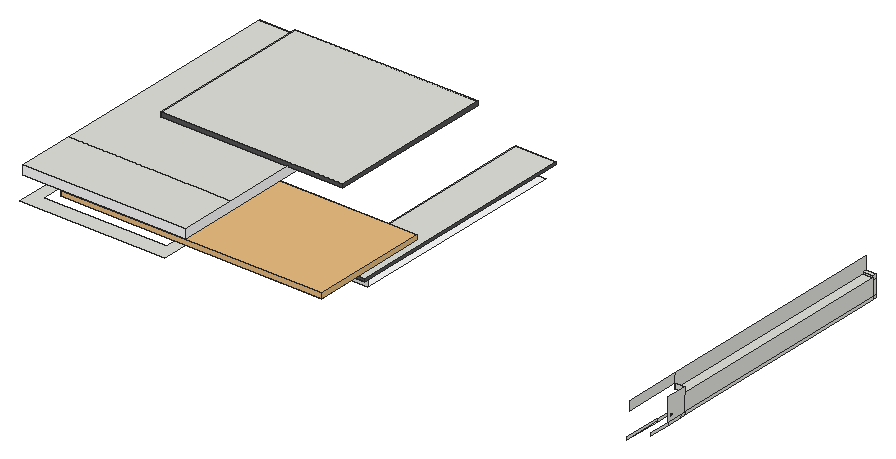
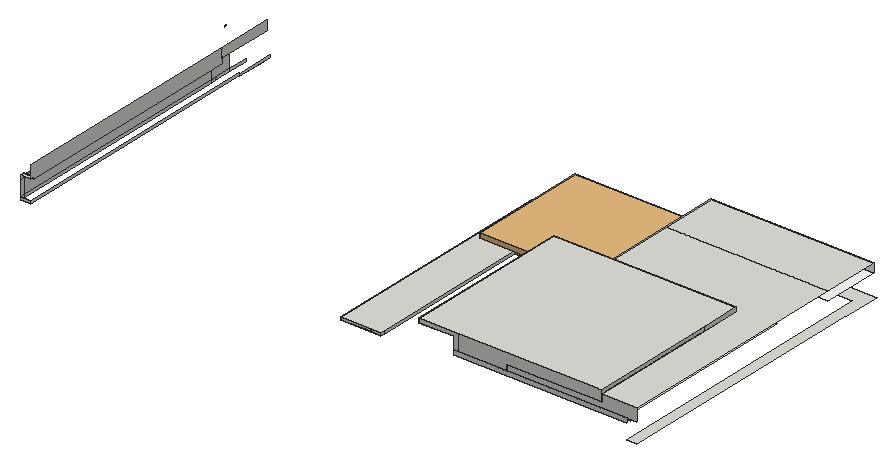
# SketchUp Ruby script. Lengths in inches.
U = 1.inch
M = Sketchup.active_model
def pt(a) = Geom::Point3d.new(a.map { |v| v * U })
def face(e, loops, mat)
  f = e.add_face(loops[0].map { |a| pt(a) })
  loops[1..].each { |l| e.add_face(l.map { |a| pt(a) }).erase! }
  f.material = f.back_material = mat if mat
  f
end
# faces: each face lists its corners as indices into pts; further lists are holes
def faces(e, pts, list, mat = nil) = list.each { |f| face(e, (f[0].is_a?(Array) ? f : [f]).map { |l| l.map { |i| pts[i] } }, mat) }
# xy, xz, yz: faces in a plane at the given z, y or x. An outline is a flat list of corners, or four numbers for a rectangle; further outlines are holes
def ring(l) = l.size == 4 ? [[l[0], l[1]], [l[2], l[1]], [l[2], l[3]], [l[0], l[3]]] : l.each_slice(2).to_a
def flat(e, list, mat, &to3) = list.each { |f| face(e, (f[0].is_a?(Array) ? f : [f]).map { |l| ring(l).map { |u, v| to3.(u, v) } }, mat) }
def xy(e, z, list, mat = nil) = flat(e, list, mat) { |x, y| [x, y, z] }
def xz(e, y, list, mat = nil) = flat(e, list, mat) { |x, z| [x, y, z] }
def yz(e, x, list, mat = nil) = flat(e, list, mat) { |y, z| [x, y, z] }
def lines(e, pts, list) = list.each { |a, b| e.add_line(pt(pts[a]), pt(pts[b])) }
# prism: a flat outline (further loops are holes) pulled along v
def prism(e, loops, v, mat = nil)
  f = face(e, loops, mat); d = Geom::Vector3d.new(v.map { |x| x * U })
  f.pushpull(f.normal.samedirection?(d) ? d.length : -d.length)
end
def box(e, o, s, mat = nil) = prism(e, [[o, [o[0] + s[0], o[1], o[2]], [o[0] + s[0], o[1] + s[1], o[2]], [o[0], o[1] + s[1], o[2]]]], [0, 0, s[2]], mat)
def at(x, y, z, deg = 0) = Geom::Transformation.translation(pt([x, y, z])) * Geom::Transformation.rotation(ORIGIN, Z_AXIS, deg.degrees)
def axes(o, x, y, z) = Geom::Transformation.new([*x, 0, *y, 0, *z, 0, *pt(o).to_a, 1])
def part(name) = M.definitions.add(name)
# library, detail: a bought-in or finely detailed component or shape, given as its bounding box
def library(name, o, s) = part(name).tap { |d| box(d.entities, o, s) }
def detail(e, o, s) = box(e.add_group.entities, o, s)
def put(e, d, t, mat = nil) = e.add_instance(d, t).tap { |i| i.material = mat if mat }
def group(e, t, mat = nil) = e.add_group.tap { |g| g.transformation = t; g.material = mat if mat }.entities
root = M.entities
M.materials.add("[Color M00]").color = [255, 255, 255]
M.materials.add("[Color M06]").color = [86, 86, 86]
c1 = library("Mesh Light\#4",[-0.5,-0.5,-0.1],[1,1,0.2])
c2 = part("Group\#24")
xy(c2.entities,0,[[203.13,95.41,201.58,95.62,200.13,96.22,198.89,97.17,197.9375,98.41,197.34,99.86,197.13,101.41,197.34,102.96,197.9375,104.41,198.89,105.65,200.13,106.61,201.58,107.21,203.13,107.41,204.6875,107.21,206.13,106.61,207.375,105.65,208.33,104.41,208.93,102.96,209.13,101.41,208.93,99.86,208.33,98.41,207.375,97.17,206.13,96.22,204.6875,95.62],[281.57,95.41,280.02,95.62,278.57,96.22,277.33,97.17,276.375,98.41,275.77,99.86,275.57,101.41,275.77,102.96,276.375,104.41,277.33,105.65,278.57,106.61,280.02,107.21,281.57,107.41,283.125,107.21,284.57,106.61,285.8125,105.65,286.77,104.41,287.37,102.96,287.57,101.41,287.37,99.86,286.77,98.41,285.8125,97.17,284.57,96.22,283.125,95.62],[350.95,95.41,349.39,95.62,347.95,96.22,346.7,97.17,345.75,98.41,345.15,99.86,344.95,101.41,345.15,102.96,345.75,104.41,346.7,105.65,347.95,106.61,349.39,107.21,350.95,107.41,352.5,107.21,353.95,106.61,355.1875,105.65,356.14,104.41,356.74,102.96,356.95,101.41,356.74,99.86,356.14,98.41,355.1875,97.17,353.95,96.22,352.5,95.62],[376,162.85,374.44,163.05,373,163.65,371.75,164.6,370.8,165.85,370.2,167.29,370,168.85,370.2,170.4,370.8,171.85,371.75,173.09,373,174.04,374.44,174.64,376,174.85,377.55,174.64,379,174.04,380.24,173.09,381.19,171.85,381.79,170.4,382,168.85,381.79,167.29,381.19,165.85,380.24,164.6,379,163.65,377.55,163.05]],"[Color M00]")
xy(c2.entities,33.4375,[[6,0,4.45,0.2,3,0.8,1.76,1.76,0.8,3,0.2,4.45,0,6,0.2,7.55,0.8,9,1.76,10.24,3,11.2,4.45,11.8,6,12,7.55,11.8,9,11.2,10.24,10.24,11.2,9,11.8,7.55,12,6,11.8,4.45,11.2,3,10.24,1.76,9,0.8,7.55,0.2],[83.125,0,81.57,0.2,80.125,0.8,78.88,1.76,77.93,3,77.33,4.45,77.125,6,77.33,7.55,77.93,9,78.88,10.24,80.125,11.2,81.57,11.8,83.125,12,84.68,11.8,86.125,11.2,87.37,10.24,88.32,9,88.92,7.55,89.125,6,88.92,4.45,88.32,3,87.37,1.76,86.125,0.8,84.68,0.2],[166.6875,0,165.13,0.2,163.6875,0.8,162.44,1.76,161.49,3,160.89,4.45,160.6875,6,160.89,7.55,161.49,9,162.44,10.24,163.6875,11.2,165.13,11.8,166.6875,12,168.24,11.8,169.6875,11.2,170.93,10.24,171.88,9,172.48,7.55,172.6875,6,172.48,4.45,171.88,3,170.93,1.76,169.6875,0.8,168.24,0.2],[166.6875,88.9375,165.13,89.14,163.6875,89.74,162.44,90.69,161.49,91.9375,160.89,93.38,160.6875,94.9375,160.89,96.49,161.49,97.9375,162.44,99.18,163.6875,100.13,165.13,100.73,166.6875,100.9375,168.24,100.73,169.6875,100.13,170.93,99.18,171.88,97.9375,172.48,96.49,172.6875,94.9375,172.48,93.38,171.88,91.9375,170.93,90.69,169.6875,89.74,168.24,89.14]],"[Color M00]")
put(c2.entities,c1,axes([191,87.42,16.72],[382.99758,0,0],[0,175.84579,0],[0,0,34.4375]))
c3 = library("Group\#23",[-0.5,-0.5,-0.1],[13,110.375,0.2])
xy(root,269.375,[[1170.95,584.06,1383.39,584.06,1383.39,676.67,1376.89,676.67,1376.89,706.17,1367.875,706.17,1367.875,607.33,1187.0625,607.33,1187.0625,1021.31,1172.33,1021.31,1172.33,638.99,1170.95,638.99],[1376.89,676.67,1383.39,731.24]])
xy(root,269.375,[[[1383.39,676.67,1383.39,731.24,1567.08,731.24,1567.08,1001.66,1607.7,1001.66,1607.7,676.67],[1497.04,698.72,1498.6,698.92,1500.04,699.52,1501.29,700.47,1502.24,701.72,1502.84,703.16,1503.04,704.72,1502.84,706.27,1502.24,707.72,1501.29,708.96,1500.04,709.91,1498.6,710.51,1497.04,710.72,1495.49,710.51,1494.04,709.91,1492.8,708.96,1491.85,707.72,1491.25,706.27,1491.04,704.72,1491.25,703.16,1491.85,701.72,1492.8,700.47,1494.04,699.52,1495.49,698.92],[1566.42,698.72,1567.97,698.92,1569.42,699.52,1570.66,700.47,1571.61,701.72,1572.21,703.16,1572.42,704.72,1572.21,706.27,1571.61,707.72,1570.66,708.96,1569.42,709.91,1567.97,710.51,1566.42,710.72,1564.86,710.51,1563.42,709.91,1562.17,708.96,1561.22,707.72,1560.62,706.27,1560.42,704.72,1560.62,703.16,1561.22,701.72,1562.17,700.47,1563.42,699.52,1564.86,698.92],[1418.61,698.72,1420.16,698.92,1421.61,699.52,1422.85,700.47,1423.8,701.72,1424.4,703.16,1424.61,704.72,1424.4,706.27,1423.8,707.72,1422.85,708.96,1421.61,709.91,1420.16,710.51,1418.61,710.72,1417.05,710.51,1415.61,709.91,1414.36,708.96,1413.41,707.72,1412.81,706.27,1412.61,704.72,1412.81,703.16,1413.41,701.72,1414.36,700.47,1415.61,699.52,1417.05,698.92],[1591.47,766.15,1593.02,766.35,1594.47,766.95,1595.71,767.91,1596.67,769.15,1597.27,770.6,1597.47,772.15,1597.27,773.7,1596.67,775.15,1595.71,776.39,1594.47,777.35,1593.02,777.95,1591.47,778.15,1589.92,777.95,1588.47,777.35,1587.23,776.39,1586.27,775.15,1585.67,773.7,1585.47,772.15,1585.67,770.6,1586.27,769.15,1587.23,767.91,1588.47,766.95,1589.92,766.35],[1591.47,846.59,1593.02,846.79,1594.47,847.39,1595.71,848.35,1596.67,849.59,1597.27,851.04,1597.47,852.59,1597.27,854.14,1596.67,855.59,1595.71,856.83,1594.47,857.78,1593.02,858.38,1591.47,858.59,1589.92,858.38,1588.47,857.78,1587.23,856.83,1586.27,855.59,1585.67,854.14,1585.47,852.59,1585.67,851.04,1586.27,849.59,1587.23,848.35,1588.47,847.39,1589.92,846.79],[1591.47,943.96,1593.02,944.17,1594.47,944.77,1595.71,945.72,1596.67,946.96,1597.27,948.41,1597.47,949.96,1597.27,951.52,1596.67,952.96,1595.71,954.21,1594.47,955.16,1593.02,955.76,1591.47,955.96,1589.92,955.76,1588.47,955.16,1587.23,954.21,1586.27,952.96,1585.67,951.52,1585.47,949.96,1585.67,948.41,1586.27,946.96,1587.23,945.72,1588.47,944.77,1589.92,944.17]]],"[Color M00]")
xy(root,270.375,[[2063.54,592.75,2064.92,636.6875]])
xy(root,279.25,[[1376.89,670.42,1607.7,676.67],[1376.89,676.67,1376.89,776.62,1548.25,776.62,1548.25,1021.31,1607.7,1021.31,1607.7,676.67]])
xy(root,282.6875,[[1376.89,670.42,1607.7,670.42,1607.7,1021.31,1548.25,1021.31,1548.25,776.62,1376.89,776.62]])
xy(root,291.125,[[1197.375,733.75,1197.375,1014.93,1364.27,1014.93,1364.27,854.49,1354.74,854.49,1354.74,733.75],[1364.27,854.49,1434.7,1014.93]])
xy(root,297.875,[[1187.0625,1014.93,1364.27,1021.31],[1364.27,1014.93,1434.7,1021.31]])
xy(root,299.625,[[2064.92,668.18,2079.65,1012.63]])
xy(root,302.5625,[[2064.92,1012.63,2079.65,1019]])
xy(root,302.8125,[[[1172.33,587.17,1172.33,670.48,1187.0625,670.48,1187.0625,639.17,1364.27,639.17,1364.27,832.12,1410.7,832.12,1410.7,587.17],[1221.47,603.3,1223.03,603.51,1224.47,604.11,1225.71,605.0625,1226.67,606.3,1227.27,607.75,1227.47,609.3,1227.27,610.86,1226.67,612.3,1225.71,613.55,1224.47,614.5,1223.03,615.1,1221.47,615.3,1219.92,615.1,1218.47,614.5,1217.23,613.55,1216.28,612.3,1215.68,610.86,1215.47,609.3,1215.68,607.75,1216.28,606.3,1217.23,605.0625,1218.47,604.11,1219.92,603.51],[1298.6,603.3,1300.15,603.51,1301.6,604.11,1302.84,605.0625,1303.79,606.3,1304.39,607.75,1304.6,609.3,1304.39,610.86,1303.79,612.3,1302.84,613.55,1301.6,614.5,1300.15,615.1,1298.6,615.3,1297.04,615.1,1295.6,614.5,1294.35,613.55,1293.4,612.3,1292.8,610.86,1292.6,609.3,1292.8,607.75,1293.4,606.3,1294.35,605.0625,1295.6,604.11,1297.04,603.51],[1382.16,692.24,1383.71,692.45,1385.16,693.05,1386.4,694,1387.36,695.24,1387.96,696.6875,1388.16,698.24,1387.96,699.8,1387.36,701.24,1386.4,702.48,1385.16,703.4375,1383.71,704.04,1382.16,704.24,1380.61,704.04,1379.16,703.4375,1377.92,702.48,1376.96,701.24,1376.36,699.8,1376.16,698.24,1376.36,696.6875,1376.96,695.24,1377.92,694,1379.16,693.05,1380.61,692.45],[1382.16,603.3,1383.71,603.51,1385.16,604.11,1386.4,605.0625,1387.36,606.3,1387.96,607.75,1388.16,609.3,1387.96,610.86,1387.36,612.3,1386.4,613.55,1385.16,614.5,1383.71,615.1,1382.16,615.3,1380.61,615.1,1379.16,614.5,1377.92,613.55,1376.96,612.3,1376.36,610.86,1376.16,609.3,1376.36,607.75,1376.96,606.3,1377.92,605.0625,1379.16,604.11,1380.61,603.51]]],"[Color M00]")
xy(root,305.625,[[1224.7,832.12,1364.27,1021.31]])
xy(root,316.0625,[[1172.33,587.17,1410.7,670.48],[1172.33,670.48,1410.7,670.48,1410.7,774.49,1224.7,774.49,1224.7,1021.31,1172.33,1021.31],[1410.7,774.49,1410.7,832.12,1440.7,832.12,1440.7,1021.31,1492.27,1021.31,1492.27,774.49]])
xy(root,321.8125,[[1224.7,774.49,1492.27,1021.31]])
xz(root,587.17,[[1172.33,302.8125,1410.7,316.0625]],"[Color M00]")
xz(root,636.6875,[[2063.54,270.375,2064.92,274.0625]])
xz(root,668.18,[[2064.92,299.625,2079.65,307.5]])
xz(root,670.42,[[1376.89,279.25,1607.7,282.6875]],"[Color M06]")
xz(root,676.67,[[1376.89,269.375,1607.7,279.25]])
xz(root,774.49,[[1224.7,316.0625,1492.27,321.8125]],"[Color M06]")
xz(root,776.62,[[1376.89,279.25,1548.25,282.6875]])
xz(root,832.12,[[1364.27,302.8125,1410.7,305.625]])
xz(root,1012.63,[[2064.92,299.625,2079.65,302.5625]])
xz(root,1014.93,[[1187.0625,291.125,1364.27,297.875],[1364.27,291.125,1434.7,297.875]])
xz(root,1019,[[2064.92,270.375,2079.65,274.0625]])
xz(root,1021.31,[[1548.25,279.25,1563.95,282.6875],[1563.95,279.25,1607.7,282.6875],[1187.0625,291.125,1440.7,297.875],[1172.33,297.875,1172.33,316.0625,1224.7,316.0625,1224.7,305.625,1364.27,305.625,1364.27,297.875],[1364.27,297.875,1364.27,305.625,1224.7,305.625,1224.7,321.8125,1434.7,321.8125,1434.7,297.875],
  [1434.7,297.875,1434.7,321.8125,1492.27,321.8125,1492.27,316.0625,1440.7,316.0625,1440.7,297.875]])
yz(root,1224.7,[[804.12,305.625,832.12,316.0625],[832.12,305.625,1021.31,316.0625],[774.49,316.0625,832.12,321.8125],[832.12,316.0625,1021.31,321.8125]])
yz(root,1364.27,[[832.12,291.125,1014.93,297.875],[832.12,297.875,1021.31,305.625]])
yz(root,1376.89,[[670.42,279.25,776.62,282.6875]])
yz(root,1410.7,[[587.17,302.8125,832.12,316.0625]],"[Color M00]")
yz(root,1492.27,[[774.49,316.0625,1021.31,321.8125]],"[Color M06]")
yz(root,1548.25,[[776.62,279.25,1014.93,282.6875],[1014.93,279.25,1021.31,282.6875]])
yz(root,1607.7,[[670.42,279.25,1021.31,282.6875]],"[Color M06]")
yz(root,2063.54,[[581.75,270.375,636.6875,274.0625]])
yz(root,2064.92,[[636.6875,270.375,1019,274.0625],[668.18,299.625,668.18,320.75,1019,320.75,1019,302.5625,1012.63,302.5625,1012.63,299.625],[584.86,307.5,668.18,320.75]])
yz(root,2079.65,[[605.03,270.375,636.86,274.0625],[636.86,270.375,660.21,274.0625],[660.21,270.375,668.18,274.0625],[668.18,270.375,1012.63,274.0625],[1012.63,270.375,1019,274.0625],
  [636.86,274.0625,668.18,307.5],[668.18,274.0625,1012.63,299.625],[1012.63,274.0625,1019,295.8125],[1012.63,295.8125,1019,302.5625]])
p = [[1418.61,698.72,269.375],[1417.05,698.92,269.375],[1417.05,698.92,270.0625],[1418.61,698.72,270.0625],[1420.16,698.92,269.375],[1420.16,698.92,270.0625],
  [1497.04,698.72,269.375],[1495.49,698.92,269.375],[1495.49,698.92,270.0625],[1497.04,698.72,270.0625],[1498.6,698.92,269.375],[1498.6,698.92,270.0625],
  [1566.42,698.72,269.375],[1564.86,698.92,269.375],[1564.86,698.92,270.0625],[1566.42,698.72,270.0625],[1567.97,698.92,269.375],[1567.97,698.92,270.0625],
  [1415.61,699.52,269.375],[1415.61,699.52,270.0625],[1421.61,699.52,269.375],[1421.61,699.52,270.0625],[1494.04,699.52,269.375],[1494.04,699.52,270.0625],
  [1500.04,699.52,269.375],[1500.04,699.52,270.0625],[1563.42,699.52,269.375],[1563.42,699.52,270.0625],[1569.42,699.52,269.375],[1569.42,699.52,270.0625],
  [1414.36,700.47,269.375],[1414.36,700.47,270.0625],[1422.85,700.47,269.375],[1422.85,700.47,270.0625],[1492.8,700.47,269.375],[1492.8,700.47,270.0625],
  [1501.29,700.47,269.375],[1501.29,700.47,270.0625],[1562.17,700.47,269.375],[1562.17,700.47,270.0625],[1570.66,700.47,269.375],[1570.66,700.47,270.0625],
  [1413.41,701.72,269.375],[1413.41,701.72,270.0625],[1423.8,701.72,269.375],[1423.8,701.72,270.0625],[1491.85,701.72,269.375],[1491.85,701.72,270.0625],
  [1502.24,701.72,269.375],[1502.24,701.72,270.0625],[1561.22,701.72,269.375],[1561.22,701.72,270.0625],[1571.61,701.72,269.375],[1571.61,701.72,270.0625],
  [1412.81,703.16,269.375],[1412.81,703.16,270.0625],[1424.4,703.16,269.375],[1424.4,703.16,270.0625],[1491.25,703.16,269.375],[1491.25,703.16,270.0625],
  [1502.84,703.16,269.375],[1502.84,703.16,270.0625],[1560.62,703.16,269.375],[1560.62,703.16,270.0625],[1572.21,703.16,269.375],[1572.21,703.16,270.0625],
  [1412.61,704.72,269.375],[1412.61,704.72,270.0625],[1424.61,704.72,269.375],[1424.61,704.72,270.0625],[1491.04,704.72,269.375],[1491.04,704.72,270.0625],
  [1503.04,704.72,269.375],[1503.04,704.72,270.0625],[1560.42,704.72,269.375],[1560.42,704.72,270.0625],[1572.42,704.72,269.375],[1572.42,704.72,270.0625],
  [1412.81,706.27,269.375],[1412.81,706.27,270.0625],[1424.4,706.27,269.375],[1424.4,706.27,270.0625],[1491.25,706.27,269.375],[1491.25,706.27,270.0625],
  [1502.84,706.27,269.375],[1502.84,706.27,270.0625],[1560.62,706.27,269.375],[1560.62,706.27,270.0625],[1572.21,706.27,269.375],[1572.21,706.27,270.0625],
  [1413.41,707.72,269.375],[1413.41,707.72,270.0625],[1423.8,707.72,269.375],[1423.8,707.72,270.0625],[1491.85,707.72,269.375],[1491.85,707.72,270.0625],
  [1502.24,707.72,269.375],[1502.24,707.72,270.0625],[1561.22,707.72,269.375],[1561.22,707.72,270.0625],[1571.61,707.72,269.375],[1571.61,707.72,270.0625],
  [1414.36,708.96,269.375],[1414.36,708.96,270.0625],[1422.85,708.96,269.375],[1422.85,708.96,270.0625],[1492.8,708.96,269.375],[1492.8,708.96,270.0625],
  [1501.29,708.96,269.375],[1501.29,708.96,270.0625],[1562.17,708.96,269.375],[1562.17,708.96,270.0625],[1570.66,708.96,269.375],[1570.66,708.96,270.0625],
  [1415.61,709.91,269.375],[1415.61,709.91,270.0625],[1421.61,709.91,269.375],[1421.61,709.91,270.0625],[1494.04,709.91,269.375],[1494.04,709.91,270.0625],
  [1500.04,709.91,269.375],[1500.04,709.91,270.0625],[1563.42,709.91,269.375],[1563.42,709.91,270.0625],[1569.42,709.91,269.375],[1569.42,709.91,270.0625],
  [1417.05,710.51,269.375],[1417.05,710.51,270.0625],[1420.16,710.51,269.375],[1420.16,710.51,270.0625],[1495.49,710.51,269.375],[1495.49,710.51,270.0625],
  [1498.6,710.51,269.375],[1498.6,710.51,270.0625],[1564.86,710.51,269.375],[1564.86,710.51,270.0625],[1567.97,710.51,269.375],[1567.97,710.51,270.0625],
  [1418.61,710.72,269.375],[1418.61,710.72,270.0625],[1497.04,710.72,269.375],[1497.04,710.72,270.0625],[1566.42,710.72,269.375],[1566.42,710.72,270.0625],
  [1591.47,766.15,269.375],[1589.92,766.35,269.375],[1589.92,766.35,270.0625],[1591.47,766.15,270.0625],[1593.02,766.35,269.375],[1593.02,766.35,270.0625],
  [1588.47,766.95,269.375],[1588.47,766.95,270.0625],[1594.47,766.95,269.375],[1594.47,766.95,270.0625],[1587.23,767.91,269.375],[1587.23,767.91,270.0625],
  [1595.71,767.91,269.375],[1595.71,767.91,270.0625],[1586.27,769.15,269.375],[1586.27,769.15,270.0625],[1596.67,769.15,269.375],[1596.67,769.15,270.0625],
  [1585.67,770.6,269.375],[1585.67,770.6,270.0625],[1597.27,770.6,269.375],[1597.27,770.6,270.0625],[1585.47,772.15,269.375],[1585.47,772.15,270.0625],
  [1597.47,772.15,269.375],[1597.47,772.15,270.0625],[1585.67,773.7,269.375],[1585.67,773.7,270.0625],[1597.27,773.7,269.375],[1597.27,773.7,270.0625],
  [1586.27,775.15,269.375],[1586.27,775.15,270.0625],[1596.67,775.15,269.375],[1596.67,775.15,270.0625],[1587.23,776.39,269.375],[1587.23,776.39,270.0625],
  [1595.71,776.39,269.375],[1595.71,776.39,270.0625],[1588.47,777.35,269.375],[1588.47,777.35,270.0625],[1594.47,777.35,269.375],[1594.47,777.35,270.0625],
  [1589.92,777.95,269.375],[1589.92,777.95,270.0625],[1593.02,777.95,269.375],[1593.02,777.95,270.0625],[1591.47,778.15,269.375],[1591.47,778.15,270.0625],
  [1591.47,846.59,269.375],[1589.92,846.79,269.375],[1589.92,846.79,270.0625],[1591.47,846.59,270.0625],[1593.02,846.79,269.375],[1593.02,846.79,270.0625],
  [1588.47,847.39,269.375],[1588.47,847.39,270.0625],[1594.47,847.39,269.375],[1594.47,847.39,270.0625],[1587.23,848.35,269.375],[1587.23,848.35,270.0625],
  [1595.71,848.35,269.375],[1595.71,848.35,270.0625],[1586.27,849.59,269.375],[1586.27,849.59,270.0625],[1596.67,849.59,269.375],[1596.67,849.59,270.0625],
  [1585.67,851.04,269.375],[1585.67,851.04,270.0625],[1597.27,851.04,269.375],[1597.27,851.04,270.0625],[1585.47,852.59,269.375],[1585.47,852.59,270.0625],
  [1597.47,852.59,269.375],[1597.47,852.59,270.0625],[1585.67,854.14,269.375],[1585.67,854.14,270.0625],[1597.27,854.14,269.375],[1597.27,854.14,270.0625],
  [1586.27,855.59,269.375],[1586.27,855.59,270.0625],[1596.67,855.59,269.375],[1596.67,855.59,270.0625],[1587.23,856.83,269.375],[1587.23,856.83,270.0625],
  [1595.71,856.83,269.375],[1595.71,856.83,270.0625],[1588.47,857.78,269.375],[1588.47,857.78,270.0625],[1594.47,857.78,269.375],[1594.47,857.78,270.0625],
  [1589.92,858.38,269.375],[1589.92,858.38,270.0625],[1593.02,858.38,269.375],[1593.02,858.38,270.0625],[1591.47,858.59,269.375],[1591.47,858.59,270.0625],
  [1591.47,943.96,269.375],[1589.92,944.17,269.375],[1589.92,944.17,270.0625],[1591.47,943.96,270.0625],[1593.02,944.17,269.375],[1593.02,944.17,270.0625],
  [1588.47,944.77,269.375],[1588.47,944.77,270.0625],[1594.47,944.77,269.375],[1594.47,944.77,270.0625],[1587.23,945.72,269.375],[1587.23,945.72,270.0625],
  [1595.71,945.72,269.375],[1595.71,945.72,270.0625],[1586.27,946.96,269.375],[1586.27,946.96,270.0625],[1596.67,946.96,269.375],[1596.67,946.96,270.0625],
  [1585.67,948.41,269.375],[1585.67,948.41,270.0625],[1597.27,948.41,269.375],[1597.27,948.41,270.0625],[1585.47,949.96,269.375],[1585.47,949.96,270.0625],
  [1597.47,949.96,269.375],[1597.47,949.96,270.0625],[1585.67,951.52,269.375],[1585.67,951.52,270.0625],[1597.27,951.52,269.375],[1597.27,951.52,270.0625],
  [1586.27,952.96,269.375],[1586.27,952.96,270.0625],[1596.67,952.96,269.375],[1596.67,952.96,270.0625],[1587.23,954.21,269.375],[1587.23,954.21,270.0625],
  [1595.71,954.21,269.375],[1595.71,954.21,270.0625],[1588.47,955.16,269.375],[1588.47,955.16,270.0625],[1594.47,955.16,269.375],[1594.47,955.16,270.0625],
  [1589.92,955.76,269.375],[1589.92,955.76,270.0625],[1593.02,955.76,269.375],[1593.02,955.76,270.0625],[1591.47,955.96,269.375],[1591.47,955.96,270.0625],
  [1221.47,603.3,302.8125],[1219.92,603.51,302.8125],[1219.92,603.51,303.5],[1221.47,603.3,303.5],[1223.03,603.51,302.8125],[1223.03,603.51,303.5],
  [1298.6,603.3,302.8125],[1297.04,603.51,302.8125],[1297.04,603.51,303.5],[1298.6,603.3,303.5],[1300.15,603.51,302.8125],[1300.15,603.51,303.5],
  [1382.16,603.3,302.8125],[1380.61,603.51,302.8125],[1380.61,603.51,303.5],[1382.16,603.3,303.5],[1383.71,603.51,302.8125],[1383.71,603.51,303.5],
  [1218.47,604.11,302.8125],[1218.47,604.11,303.5],[1224.47,604.11,302.8125],[1224.47,604.11,303.5],[1295.6,604.11,302.8125],[1295.6,604.11,303.5],
  [1301.6,604.11,302.8125],[1301.6,604.11,303.5],[1379.16,604.11,302.8125],[1379.16,604.11,303.5],[1385.16,604.11,302.8125],[1385.16,604.11,303.5],
  [1217.23,605.0625,302.8125],[1217.23,605.0625,303.5],[1225.71,605.0625,302.8125],[1225.71,605.0625,303.5],[1294.35,605.0625,302.8125],[1294.35,605.0625,303.5],
  [1302.84,605.0625,302.8125],[1302.84,605.0625,303.5],[1377.92,605.0625,302.8125],[1377.92,605.0625,303.5],[1386.4,605.0625,302.8125],[1386.4,605.0625,303.5],
  [1216.28,606.3,302.8125],[1216.28,606.3,303.5],[1226.67,606.3,302.8125],[1226.67,606.3,303.5],[1293.4,606.3,302.8125],[1293.4,606.3,303.5],
  [1303.79,606.3,302.8125],[1303.79,606.3,303.5],[1376.96,606.3,302.8125],[1376.96,606.3,303.5],[1387.36,606.3,302.8125],[1387.36,606.3,303.5],
  [1215.68,607.75,302.8125],[1215.68,607.75,303.5],[1227.27,607.75,302.8125],[1227.27,607.75,303.5],[1292.8,607.75,302.8125],[1292.8,607.75,303.5],
  [1304.39,607.75,302.8125],[1304.39,607.75,303.5],[1376.36,607.75,302.8125],[1376.36,607.75,303.5],[1387.96,607.75,302.8125],[1387.96,607.75,303.5],
  [1227.47,609.3,302.8125],[1227.47,609.3,303.5],[1292.6,609.3,302.8125],[1292.6,609.3,303.5],[1304.6,609.3,302.8125],[1304.6,609.3,303.5],
  [1376.16,609.3,302.8125],[1376.16,609.3,303.5],[1388.16,609.3,302.8125],[1388.16,609.3,303.5],[1215.47,609.3,302.8125],[1215.68,610.86,302.8125],
  [1215.68,610.86,303.5],[1215.47,609.3,303.5],[1227.27,610.86,302.8125],[1227.27,610.86,303.5],[1292.8,610.86,302.8125],[1292.8,610.86,303.5],
  [1304.39,610.86,302.8125],[1304.39,610.86,303.5],[1376.36,610.86,302.8125],[1376.36,610.86,303.5],[1387.96,610.86,302.8125],[1387.96,610.86,303.5],
  [1216.28,612.3,302.8125],[1216.28,612.3,303.5],[1226.67,612.3,302.8125],[1226.67,612.3,303.5],[1293.4,612.3,302.8125],[1293.4,612.3,303.5],
  [1303.79,612.3,302.8125],[1303.79,612.3,303.5],[1376.96,612.3,302.8125],[1376.96,612.3,303.5],[1387.36,612.3,302.8125],[1387.36,612.3,303.5],
  [1217.23,613.55,302.8125],[1217.23,613.55,303.5],[1225.71,613.55,302.8125],[1225.71,613.55,303.5],[1294.35,613.55,302.8125],[1294.35,613.55,303.5],
  [1302.84,613.55,302.8125],[1302.84,613.55,303.5],[1377.92,613.55,302.8125],[1377.92,613.55,303.5],[1386.4,613.55,302.8125],[1386.4,613.55,303.5],
  [1218.47,614.5,302.8125],[1218.47,614.5,303.5],[1224.47,614.5,302.8125],[1224.47,614.5,303.5],[1295.6,614.5,302.8125],[1295.6,614.5,303.5],
  [1301.6,614.5,302.8125],[1301.6,614.5,303.5],[1379.16,614.5,302.8125],[1379.16,614.5,303.5],[1385.16,614.5,302.8125],[1385.16,614.5,303.5],
  [1219.92,615.1,302.8125],[1219.92,615.1,303.5],[1223.03,615.1,302.8125],[1223.03,615.1,303.5],[1297.04,615.1,302.8125],[1297.04,615.1,303.5],
  [1300.15,615.1,302.8125],[1300.15,615.1,303.5],[1380.61,615.1,302.8125],[1380.61,615.1,303.5],[1383.71,615.1,302.8125],[1383.71,615.1,303.5],
  [1221.47,615.3,302.8125],[1221.47,615.3,303.5],[1298.6,615.3,302.8125],[1298.6,615.3,303.5],[1382.16,615.3,302.8125],[1382.16,615.3,303.5],
  [1382.16,692.24,302.8125],[1380.61,692.45,302.8125],[1380.61,692.45,303.5],[1382.16,692.24,303.5],[1383.71,692.45,302.8125],[1383.71,692.45,303.5],
  [1379.16,693.05,302.8125],[1379.16,693.05,303.5],[1385.16,693.05,302.8125],[1385.16,693.05,303.5],[1377.92,694,302.8125],[1377.92,694,303.5],
  [1386.4,694,302.8125],[1386.4,694,303.5],[1376.96,695.24,302.8125],[1376.96,695.24,303.5],[1387.36,695.24,302.8125],[1387.36,695.24,303.5],
  [1376.36,696.6875,302.8125],[1376.36,696.6875,303.5],[1387.96,696.6875,302.8125],[1387.96,696.6875,303.5],[1376.16,698.24,302.8125],[1376.16,698.24,303.5],
  [1388.16,698.24,302.8125],[1388.16,698.24,303.5],[1376.36,699.8,302.8125],[1376.36,699.8,303.5],[1387.96,699.8,302.8125],[1387.96,699.8,303.5],
  [1376.96,701.24,302.8125],[1376.96,701.24,303.5],[1387.36,701.24,302.8125],[1387.36,701.24,303.5],[1377.92,702.48,302.8125],[1377.92,702.48,303.5],
  [1386.4,702.48,302.8125],[1386.4,702.48,303.5],[1379.16,703.4375,302.8125],[1379.16,703.4375,303.5],[1385.16,703.4375,302.8125],[1385.16,703.4375,303.5],
  [1380.61,704.04,302.8125],[1380.61,704.04,303.5],[1383.71,704.04,302.8125],[1383.71,704.04,303.5],[1382.16,704.24,302.8125],[1382.16,704.24,303.5],
  [2108.27,605.45,307.5],[2108.0625,607,307.5],[2108.0625,607,308.1875],[2108.27,605.45,308.1875],[2108.27,608.55,307.5],[2108.27,608.55,308.1875],
  [2089.96,731.45,295.8125],[2079.65,731.45,295.8125],[1224.7,804.12,305.625],[1394.33,804.12,305.625],[1434.7,1014.93,297.875],[1434.7,832.12,297.875],
  [1434.7,854.49,291.125],[1440.7,854.49,291.125],[1567.08,1001.66,269.375],[1567.08,1001.66,277.5],[1434.7,832.12,291.125]]
faces(root,p,[[0,1,2,3],[4,0,3,5],[6,7,8,9],[10,6,9,11],[12,13,14,15],[16,12,15,17],[1,18,19,2],[20,4,5,21],
  [7,22,23,8],[24,10,11,25],[13,26,27,14],[28,16,17,29],[18,30,31,19],[32,20,21,33],[22,34,35,23],[36,24,25,37],
  [26,38,39,27],[40,28,29,41],[30,42,43,31],[44,32,33,45],[34,46,47,35],[48,36,37,49],[38,50,51,39],[52,40,41,53],
  [42,54,55,43],[56,44,45,57],[46,58,59,47],[60,48,49,61],[50,62,63,51],[64,52,53,65],[54,66,67,55],[68,56,57,69],
  [58,70,71,59],[72,60,61,73],[62,74,75,63],[76,64,65,77],[66,78,79,67],[80,68,69,81],[70,82,83,71],[84,72,73,85],
  [74,86,87,75],[88,76,77,89],[78,90,91,79],[92,80,81,93],[82,94,95,83],[96,84,85,97],[86,98,99,87],[100,88,89,101],
  [90,102,103,91],[104,92,93,105],[94,106,107,95],[108,96,97,109],[98,110,111,99],[112,100,101,113],[102,114,115,103],[116,104,105,117],
  [106,118,119,107],[120,108,109,121],[110,122,123,111],[124,112,113,125],[114,126,127,115],[128,116,117,129],[118,130,131,119],[132,120,121,133],
  [122,134,135,123],[136,124,125,137],[126,138,139,127],[138,128,129,139],[130,140,141,131],[140,132,133,141],[134,142,143,135],[142,136,137,143],
  [144,145,146,147],[148,144,147,149],[145,150,151,146],[152,148,149,153],[150,154,155,151],[156,152,153,157],[154,158,159,155],[160,156,157,161],
  [158,162,163,159],[164,160,161,165],[162,166,167,163],[168,164,165,169],[166,170,171,167],[172,168,169,173],[170,174,175,171],[176,172,173,177],
  [174,178,179,175],[180,176,177,181],[178,182,183,179],[184,180,181,185],[182,186,187,183],[188,184,185,189],[186,190,191,187],[190,188,189,191],
  [192,193,194,195],[196,192,195,197],[193,198,199,194],[200,196,197,201],[198,202,203,199],[204,200,201,205],[202,206,207,203],[208,204,205,209],
  [206,210,211,207],[212,208,209,213],[210,214,215,211],[216,212,213,217],[214,218,219,215],[220,216,217,221],[218,222,223,219],[224,220,221,225],
  [222,226,227,223],[228,224,225,229],[226,230,231,227],[232,228,229,233],[230,234,235,231],[236,232,233,237],[234,238,239,235],[238,236,237,239],
  [240,241,242,243],[244,240,243,245],[241,246,247,242],[248,244,245,249],[246,250,251,247],[252,248,249,253],[250,254,255,251],[256,252,253,257],
  [254,258,259,255],[260,256,257,261],[258,262,263,259],[264,260,261,265],[262,266,267,263],[268,264,265,269],[266,270,271,267],[272,268,269,273],
  [270,274,275,271],[276,272,273,277],[274,278,279,275],[280,276,277,281],[278,282,283,279],[284,280,281,285],[282,286,287,283],[286,284,285,287],
  [288,289,290,291],[292,288,291,293],[294,295,296,297],[298,294,297,299],[300,301,302,303],[304,300,303,305],[289,306,307,290],[308,292,293,309],
  [295,310,311,296],[312,298,299,313],[301,314,315,302],[316,304,305,317],[306,318,319,307],[320,308,309,321],[310,322,323,311],[324,312,313,325],
  [314,326,327,315],[328,316,317,329],[318,330,331,319],[332,320,321,333],[322,334,335,323],[336,324,325,337],[326,338,339,327],[340,328,329,341],
  [330,342,343,331],[344,332,333,345],[334,346,347,335],[348,336,337,349],[338,350,351,339],[352,340,341,353],[354,344,345,355],[346,356,357,347],
  [358,348,349,359],[350,360,361,351],[362,352,353,363],[364,365,366,367],[368,354,355,369],[356,370,371,357],[372,358,359,373],[360,374,375,361],
  [376,362,363,377],[365,378,379,366],[380,368,369,381],[370,382,383,371],[384,372,373,385],[374,386,387,375],[388,376,377,389],[378,390,391,379],
  [392,380,381,393],[382,394,395,383],[396,384,385,397],[386,398,399,387],[400,388,389,401],[390,402,403,391],[404,392,393,405],[394,406,407,395],
  [408,396,397,409],[398,410,411,399],[412,400,401,413],[402,414,415,403],[416,404,405,417],[406,418,419,407],[420,408,409,421],[410,422,423,411],
  [424,412,413,425],[414,426,427,415],[426,416,417,427],[418,428,429,419],[428,420,421,429],[422,430,431,423],[430,424,425,431],[432,433,434,435],
  [436,432,435,437],[433,438,439,434],[440,436,437,441],[438,442,443,439],[444,440,441,445],[442,446,447,443],[448,444,445,449],[446,450,451,447],
  [452,448,449,453],[450,454,455,451],[456,452,453,457],[454,458,459,455],[460,456,457,461],[458,462,463,459],[464,460,461,465],[462,466,467,463],
  [468,464,465,469],[466,470,471,467],[472,468,469,473],[470,474,475,471],[476,472,473,477],[474,478,479,475],[478,476,477,479],[480,481,482,483],
  [481,484,485,482]],"[Color M00]")
lines(root,p,[[486,487],[488,489],[490,491],[492,493],[494,495],[492,496]])
put(root,c2,at(1215.47,603.3,270.0625))
put(root,c3,at(1585.47,846.59,270.0625))
